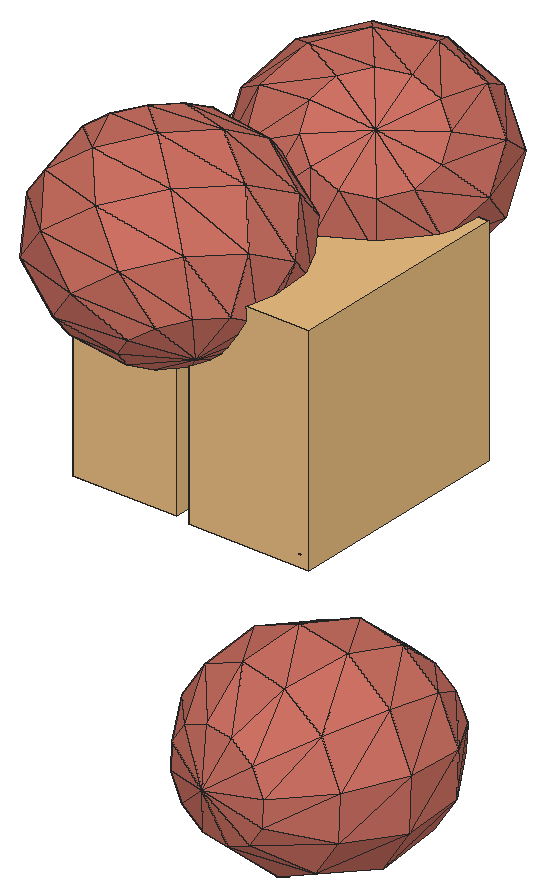
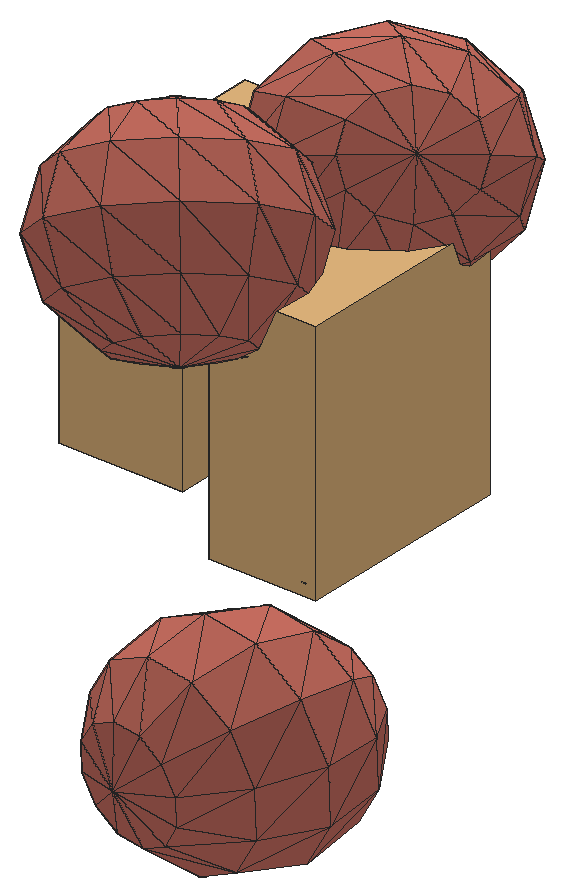
# SketchUp Ruby script. Lengths in inches.
U = 1.inch
M = Sketchup.active_model
def pt(a) = Geom::Point3d.new(a.map { |v| v * U })
def face(e, loops, mat)
  f = e.add_face(loops[0].map { |a| pt(a) })
  loops[1..].each { |l| e.add_face(l.map { |a| pt(a) }).erase! }
  f.material = f.back_material = mat if mat
  f
end
# faces: each face lists its corners as indices into pts; further lists are holes
def faces(e, pts, list, mat = nil) = list.each { |f| face(e, (f[0].is_a?(Array) ? f : [f]).map { |l| l.map { |i| pts[i] } }, mat) }
# xy, xz, yz: faces in a plane at the given z, y or x. An outline is a flat list of corners, or four numbers for a rectangle; further outlines are holes
def ring(l) = l.size == 4 ? [[l[0], l[1]], [l[2], l[1]], [l[2], l[3]], [l[0], l[3]]] : l.each_slice(2).to_a
def flat(e, list, mat, &to3) = list.each { |f| face(e, (f[0].is_a?(Array) ? f : [f]).map { |l| ring(l).map { |u, v| to3.(u, v) } }, mat) }
def xy(e, z, list, mat = nil) = flat(e, list, mat) { |x, y| [x, y, z] }
def xz(e, y, list, mat = nil) = flat(e, list, mat) { |x, z| [x, y, z] }
def yz(e, x, list, mat = nil) = flat(e, list, mat) { |y, z| [x, y, z] }
def lines(e, pts, list) = list.each { |a, b| e.add_line(pt(pts[a]), pt(pts[b])) }
# prism: a flat outline (further loops are holes) pulled along v
def prism(e, loops, v, mat = nil)
  f = face(e, loops, mat); d = Geom::Vector3d.new(v.map { |x| x * U })
  f.pushpull(f.normal.samedirection?(d) ? d.length : -d.length)
end
def box(e, o, s, mat = nil) = prism(e, [[o, [o[0] + s[0], o[1], o[2]], [o[0] + s[0], o[1] + s[1], o[2]], [o[0], o[1] + s[1], o[2]]]], [0, 0, s[2]], mat)
def at(x, y, z, deg = 0) = Geom::Transformation.translation(pt([x, y, z])) * Geom::Transformation.rotation(ORIGIN, Z_AXIS, deg.degrees)
def axes(o, x, y, z) = Geom::Transformation.new([*x, 0, *y, 0, *z, 0, *pt(o).to_a, 1])
def part(name) = M.definitions.add(name)
# library, detail: a bought-in or finely detailed component or shape, given as its bounding box
def library(name, o, s) = part(name).tap { |d| box(d.entities, o, s) }
def detail(e, o, s) = box(e.add_group.entities, o, s)
def put(e, d, t, mat = nil) = e.add_instance(d, t).tap { |i| i.material = mat if mat }
def group(e, t, mat = nil) = e.add_group.tap { |g| g.transformation = t; g.material = mat if mat }.entities
root = M.entities
M.materials.add("green").color = [174, 139, 102]
M.materials.add("vio").color = [206, 114, 100]
c1 = library("3DGeom~152_Defintion",[-440.97,-500,-219.08],[881.94,1000,438.17])
c2 = part("3DGeom~153_Defintion")
p = [[-380.69,-485.53,-210.54],[-411.26,-467,-218.1875],[-394.16,-475.51,-219.08],[-380.69,-485.53,-210.54],[-434.74,-476.74,-157.14],[-411.26,-467,-218.1875],
  [-438.29,-462.61,-191.49],[-411.26,-467,-218.1875],[-438.29,-462.61,-191.49],[-427.41,-462.28,-208.09],[-377.14,-499.67,-176.1875],[-434.74,-476.74,-157.14],
  [-380.69,-485.53,-210.54],[-377.14,-499.67,-176.1875],[-380.69,-485.53,-210.54],[-374.46,-494.375,-194.84],[-434.74,-476.74,-157.14],[-440.97,-467.9,-172.84],
  [-438.29,-462.61,-191.49],[-404.17,-495.28,-149.49],[-377.14,-499.67,-176.1875],[-388.02,-500,-159.59],[-404.17,-495.28,-149.49],[-434.74,-476.74,-157.14],
  [-404.17,-495.28,-149.49],[-421.27,-486.76,-148.59],[402.51,492.03,208.37],[431.04,458.58,149.1],[419.28,470.25,140.95],[402.51,492.03,208.37],
  [419.28,470.25,140.95],[406.85,483.28,142.92],[402.51,492.03,208.37],[406.85,483.28,142.92],[397.08,494.16,154.49],[402.51,492.03,208.37],
  [438.98,451.39,165.19],[431.04,458.58,149.1],[402.51,492.03,208.37],[397.08,494.16,154.49],[392.58,500,172.55],[402.51,492.03,208.37],
  [440.97,450.61,184.92],[438.98,451.39,165.19],[402.51,492.03,208.37],[392.58,500,172.55],[394.57,499.22,192.28],[402.51,492.03,208.37],
  [436.48,456.44,202.98],[440.97,450.61,184.92],[402.51,492.03,208.37],[426.7,467.33,214.55],[402.51,492.03,208.37],[414.27,480.36,216.53],
  [426.7,467.33,214.55]]
faces(c2.entities,p,[[0,1,2],[3,4,5],[5,4,6],[7,8,9],[10,11,12],[13,14,15],[16,17,18],[19,20,21],
  [22,11,10],[23,24,25],[26,27,28],[29,30,31],[32,33,34],[35,36,37],[38,39,40],[41,42,43],
  [44,45,46],[47,48,49],[50,51,48],[52,53,54]],"green")
c3 = part("3DGeom~238_Defintion")
p = [[47.04,-55.62,-493.71],[-13.56,-317.59,-331.8],[-140.27,-151.99,-445.55],[202.73,-206.32,-387.4],[187.3,88.625,-451.96],[-121.25,109.98,-467.72],
  [-40.27,193.26,-443.62],[-229.4,54.34,-439.92],[-257.06,246.11,-316.41],[364.69,-39.76,-339.2],[242.94,242.1,-331.5],[-8.15,281.87,-374.07],
  [-226.21,-343.77,-187.29],[-324.43,-174.66,-320.41],[-335.72,41.26,-367.67],[202.73,-206.32,-387.4],[116.79,-398.1,-129.14],[-13.56,-317.59,-331.8],
  [202.73,-206.32,-387.4],[304.09,-301.73,-177.3],[364.69,-39.76,-339.2],[304.09,-301.73,-177.3],[202.73,-206.32,-387.4],[-33.49,352.06,-277.72],
  [242.94,242.1,-331.5],[-8.15,281.87,-374.07],[-33.49,352.06,-277.72],[-335.72,41.26,-367.67],[-324.43,-174.66,-320.41],[-456.1,-117.55,-151.8],
  [-335.72,41.26,-367.67],[-411.74,74.22,-270.32],[-335.72,41.26,-367.67],[-257.06,246.11,-316.41],[364.69,-39.76,-339.2],[444.36,-157.49,-135.55],
  [304.09,-301.73,-177.3],[428.9375,137.45,-200.11],[364.69,-39.76,-339.2],[428.9375,137.45,-200.11],[-13.56,-317.59,-331.8],[-67.38,-420.77,-4],
  [-226.21,-343.77,-187.29],[-13.56,-317.59,-331.8],[199.05,363.67,-164.61],[428.9375,137.45,-200.11],[242.94,242.1,-331.5],[-33.49,352.06,-277.72],
  [199.05,363.67,-164.61],[242.94,242.1,-331.5],[-324.43,-174.66,-320.41],[-226.21,-343.77,-187.29],[-378.25,-277.83,7.4],[-324.43,-174.66,-320.41],
  [-437.09,144.42,-173.96],[-257.06,246.11,-316.41],[-404.96,233.02,-104.42],[-257.06,246.11,-316.41],[-323.98,316.3,-80.32],[-257.06,246.11,-316.41],
  [-323.98,316.3,-80.32],[-215.84,371.9375,-108.12],[-257.06,246.11,-316.41],[-109.51,385.02,-180.37],[-33.49,352.06,-277.72],[-257.06,246.11,-316.41],
  [-257.06,246.11,-316.41],[-33.49,352.06,-277.72],[-500,4.02,15.09],[428.9375,137.45,-200.11],[500,-4.02,-15.09],[378.25,277.83,-7.4],
  [428.9375,137.45,-200.11],[199.05,363.67,-164.61],[428.9375,137.45,-200.11],[-226.21,-343.77,-187.29],[-199.05,-363.67,164.61],[-226.21,-343.77,-187.29],
  [-199.05,-363.67,164.61],[-378.25,-277.83,7.4],[67.38,420.77,4],[215.84,-371.9375,108.12],[323.98,-316.3,80.32],[323.98,-316.3,80.32],
  [304.09,-301.73,-177.3],[-444.36,157.49,135.55],[378.25,277.83,-7.4],[-428.9375,-137.45,200.11],[404.96,-233.02,104.42],[323.98,-316.3,80.32],
  [109.51,-385.02,180.37],[-116.78,398.1,129.14],[-304.09,301.73,177.3],[-304.09,301.73,177.3],[-323.98,316.3,-80.32],[-304.09,301.73,177.3],
  [437.09,-144.42,173.96],[456.1,117.55,151.8],[226.21,343.77,187.29],[226.21,343.77,187.29],[378.25,277.83,-7.4],[33.49,-352.06,277.72],
  [-199.05,-363.67,164.61],[-199.05,-363.67,164.61],[-242.94,-242.09,331.5],[-242.94,-242.09,331.5],[-364.69,39.76,339.2],[257.06,-246.11,316.41],
  [323.98,-316.3,80.32],[257.06,-246.11,316.41],[257.06,-246.11,316.41],[13.56,317.59,331.8],[-202.73,206.32,387.4],[-202.73,206.32,387.4],
  [-304.09,301.73,177.3],[411.74,-74.22,270.32],[324.43,174.66,320.41],[226.21,343.77,187.29],[-199.05,-363.67,164.61],[8.15,-281.87,374.07],
  [-242.94,-242.09,331.5],[-199.05,-363.67,164.61],[8.15,-281.87,374.07],[257.06,-246.11,316.41],[-202.73,206.32,387.4],[13.56,317.59,331.8],
  [324.43,174.66,320.41],[226.21,343.77,187.29],[-428.9375,-137.45,200.11],[-242.94,-242.09,331.5],[-187.3,-88.625,451.96],[-428.9375,-137.45,200.11],
  [-364.69,39.76,339.2],[335.72,-41.26,367.67],[257.06,-246.11,316.41],[8.15,-281.87,374.07],[33.49,-352.06,277.72],[257.06,-246.11,316.41],
  [40.27,-193.26,443.62],[257.06,-246.11,316.41],[121.25,-109.98,467.72],[257.06,-246.11,316.41],[229.4,-54.34,439.92],[257.06,-246.11,316.41],
  [335.72,-41.26,367.67],[257.06,-246.11,316.41],[140.27,151.99,445.55],[335.72,-41.26,367.67],[324.43,174.66,320.41],[13.56,317.59,331.8],
  [324.43,174.66,320.41],[-202.73,206.32,387.4],[13.56,317.59,331.8],[-364.69,39.76,339.2],[-47.04,55.62,493.71],[-364.69,39.76,339.2],
  [-202.73,206.32,387.4],[335.72,-41.26,367.67],[-202.73,206.32,387.4]]
faces(c3.entities,p,[[0,1,2],[0,3,1],[4,3,0],[5,0,2],[6,0,5],[6,4,0],[5,2,7],[5,7,8],
  [6,5,8],[4,9,3],[10,9,4],[11,4,6],[11,10,4],[2,12,13],[2,1,12],[7,2,13],
  [11,6,8],[7,13,14],[7,14,8],[15,16,17],[18,19,16],[20,21,22],[23,24,25],[26,11,8],
  [27,28,29],[30,29,31],[32,31,33],[34,35,36],[37,35,38],[10,39,9],[40,41,42],[43,16,41],
  [44,45,46],[47,48,49],[50,51,52],[53,52,29],[31,54,55],[54,56,57],[56,58,59],[60,61,62],
  [63,64,65],[61,63,66],[63,48,67],[31,29,68],[31,68,54],[69,70,35],[71,70,72],[73,71,74],
  [75,41,76],[77,78,79],[63,80,48],[61,80,63],[19,81,16],[19,82,81],[35,83,84],[54,68,85],
  [54,85,56],[80,86,48],[29,52,87],[29,87,68],[35,88,89],[70,88,35],[16,90,41],[16,81,90],
  [60,91,61],[61,91,80],[56,85,92],[56,93,94],[60,95,91],[70,96,88],[97,96,70],[71,97,70],
  [98,97,71],[80,99,100],[41,101,102],[41,90,101],[91,99,80],[52,103,104],[52,105,87],[68,87,106],
  [68,106,85],[81,82,107],[108,88,109],[88,96,110],[90,81,107],[95,111,91],[91,111,99],[85,106,112],
  [85,113,114],[97,115,96],[116,115,97],[117,116,97],[118,119,120],[121,101,122],[96,115,123],[95,124,111],
  [101,90,107],[125,126,127],[128,129,130],[131,130,132],[115,133,134],[116,133,115],[135,136,137],[138,135,139],
  [140,138,141],[142,140,143],[144,142,145],[146,147,148],[149,146,150],[129,135,138],[129,138,130],[151,146,152],
  [153,130,154],[155,154,156],[146,142,157],[158,154,146],[154,140,142],[154,142,146],[130,138,140],[130,140,154]],"vio")
c4 = part("3DGeom~206_Defintion")
p = [[-12.5,-12.78,-500],[-167.87,-176.1875,-423.23],[-275,-119.8,-393.5],[139.12,-146.19,-448.74],[321.29,0,-383.61],[-198.05,84.89,-448.51],
  [146.22,154.06,-442.79],[216.18,-279.61,-308.47],[-80.33,-253.22,-393.64],[410.28,-154.06,-221.63],[410.28,-154.06,-221.63],[-373.01,-99.16,-312.41],
  [-373.01,-99.16,-312.41],[-367.81,120.64,-308.0625],[-68.03,266.84,-383.34],[-367.81,120.64,-308.0625],[-68.03,266.84,-383.34],[417.375,146.19,-215.68],
  [417.375,146.19,-215.68],[265.76,279.61,-266.94],[265.76,279.61,-266.94],[-68.03,266.84,-383.34],[-278.26,-292.39,-233.06],[-278.26,-292.39,-233.06],
  [-35.84,-330.25,-312.65],[-278.26,-292.39,-233.06],[-373.01,-99.16,-312.41],[-275,-119.8,-393.5],[-278.26,-292.39,-233.06],[494.4375,12.78,-75.41],
  [410.28,-154.06,-221.63],[321.29,0,-383.61],[321.29,0,-383.61],[417.375,146.19,-215.68],[-68.03,266.84,-383.34],[-367.81,120.64,-308.0625],
  [-264.06,308.11,-221.16],[80.21,377.28,-215.45],[-68.03,266.84,-383.34],[-264.06,308.11,-221.16],[265.76,279.61,-266.94],[-68.03,266.84,-383.34],
  [80.21,377.28,-215.45],[-35.84,-330.25,-312.65],[-46.32,-386.64,-201.97],[-278.26,-292.39,-233.06],[198.04,-377.28,-116.76],[-35.84,-330.25,-312.65],
  [198.04,-377.28,-116.76],[-35.84,-330.25,-312.65],[216.18,-279.61,-308.47],[-435.64,-119.8,-201.7],[-278.26,-292.39,-233.06],[-367.81,120.64,-308.0625],
  [389.33,-266.84,-0.27],[198.04,-377.28,-116.76],[216.18,-279.61,-308.47],[216.18,-279.61,-308.47],[-476.3,84.89,-116.29],[-264.06,308.11,-221.16],
  [401.625,253.22,10.03],[265.76,279.61,-266.94],[265.76,279.61,-266.94],[314.09,330.25,-19.5625],[314.09,330.25,-19.5625],[265.76,279.61,-266.94],
  [-108.95,-407.27,-91.25],[-206.96,-386.64,-10.17],[-314.09,-330.25,19.5625],[-314.09,-330.25,19.5625],[-401.625,-253.22,-10.03],[-278.26,-292.39,-233.06],
  [-446.12,-176.1875,-91.02],[-278.26,-292.39,-233.06],[-278.26,-292.39,-233.06],[476.3,-84.89,116.29],[-264.06,308.11,-221.16],[-389.33,266.84,0.27],
  [-89.55,413.03,-75],[-389.33,266.84,0.27],[446.12,176.1875,91.02],[206.96,386.64,10.17],[89.55,-413.03,75],[198.04,-377.28,-116.76],
  [264.06,-308.11,221.16],[198.04,-377.28,-116.76],[264.06,-308.11,221.16],[198.04,-377.28,-116.76],[389.33,-266.84,-0.27],[-494.4375,-12.78,75.41],
  [-80.21,-377.28,215.45],[435.64,119.8,201.7],[-389.33,266.84,0.27],[-198.04,377.28,116.76],[108.95,407.27,91.25],[314.09,330.25,-19.5625],
  [278.26,292.39,233.06],[278.26,292.39,233.06],[-265.76,-279.61,266.94],[-265.76,-279.61,266.94],[-417.375,-146.19,215.68],[-314.09,-330.25,19.5625],
  [-417.375,-146.19,215.68],[367.81,-120.64,308.0625],[264.06,-308.11,221.16],[367.81,-120.64,308.0625],[-410.28,154.06,221.63],[-198.04,377.28,116.76],
  [-410.28,154.06,221.63],[278.26,292.39,233.06],[-417.375,-146.19,215.68],[-314.09,-330.25,19.5625],[-265.76,-279.61,266.94],[68.03,-266.84,383.34],
  [68.03,-266.84,383.34],[264.06,-308.11,221.16],[-410.28,154.06,221.63],[-417.375,-146.19,215.68],[46.32,386.64,201.97],[278.26,292.39,233.06],
  [373.01,99.16,312.41],[367.81,-120.64,308.0625],[-198.04,377.28,116.76],[-410.28,154.06,221.63],[-216.18,279.61,308.47],[-216.18,279.61,308.47],
  [-216.18,279.61,308.47],[35.84,330.25,312.65],[35.84,330.25,312.65],[278.26,292.39,233.06],[-146.22,-154.06,442.79],[-265.76,-279.61,266.94],
  [-80.21,-377.28,215.45],[-80.21,-377.28,215.45],[68.03,-266.84,383.34],[-321.29,0,383.61],[-417.375,-146.19,215.68],[-410.28,154.06,221.63],
  [-417.375,-146.19,215.68],[-321.29,0,383.61],[198.05,-84.89,448.51],[264.06,-308.11,221.16],[367.81,-120.64,308.0625],[-216.18,279.61,308.47],
  [-410.28,154.06,221.63],[275,119.8,393.5],[167.87,176.1875,423.23],[275,119.8,393.5],[278.26,292.39,233.06],[80.33,253.22,393.64],
  [278.26,292.39,233.06],[35.84,330.25,312.65],[278.26,292.39,233.06],[275,119.8,393.5],[275,119.8,393.5],[373.01,99.16,312.41],
  [-139.12,146.19,448.74],[12.5,12.78,500],[275,119.8,393.5]]
faces(c4.entities,p,[[0,1,2],[3,1,0],[4,3,0],[0,2,5],[6,0,5],[4,0,6],[7,8,3],[9,7,3],
  [3,8,1],[10,3,4],[5,2,11],[5,12,13],[14,5,15],[6,5,16],[17,4,6],[18,6,19],
  [20,6,21],[2,1,22],[1,8,23],[8,24,25],[7,24,8],[26,27,28],[29,30,31],[29,32,33],
  [34,35,36],[37,38,39],[40,41,42],[43,44,45],[46,44,47],[48,49,50],[51,26,52],[53,26,51],
  [54,55,56],[54,57,30],[53,51,58],[59,53,58],[60,33,61],[60,62,63],[64,65,37],[66,67,45],
  [44,66,45],[67,68,45],[69,70,71],[70,72,73],[72,51,74],[75,54,30],[75,30,29],[76,58,77],
  [78,39,79],[37,39,78],[80,29,33],[80,33,60],[64,37,81],[81,37,78],[82,66,44],[82,44,83],
  [58,51,72],[84,82,85],[86,87,88],[58,72,89],[77,58,89],[90,66,82],[90,67,66],[89,72,70],
  [91,75,29],[91,29,80],[78,92,93],[94,78,93],[81,78,94],[60,95,96],[64,81,97],[98,68,67],
  [99,67,90],[100,70,101],[89,70,102],[103,104,54],[105,54,75],[77,89,106],[107,77,108],[80,60,96],
  [81,94,109],[110,111,112],[113,90,82],[114,82,115],[116,89,117],[91,80,96],[94,118,119],[94,93,118],
  [120,121,75],[120,75,91],[122,123,124],[118,93,125],[120,91,96],[118,126,127],[118,128,129],[130,131,132],
  [130,133,134],[135,136,131],[137,138,139],[140,134,141],[140,141,142],[143,144,135],[145,120,96],[146,147,148],
  [149,146,150],[151,149,152],[135,131,130],[153,140,142],[154,142,155],[143,135,156],[151,143,156],[151,156,149],
  [157,130,134],[157,134,140],[156,135,130],[146,140,158],[149,156,157],[149,157,146],[146,157,140],[156,130,157]],"vio")
c5 = part("3DGeom~199_Defintion")
p = [[-69.55,-302.43,-360.84],[-338.74,-97.12,-366.25],[-102.46,-106.03,-485.67],[189.77,-256.61,-366.85],[161.26,-86.52,-474.95],[-343.46,97.57,-361.65],
  [-107.92,118.79,-480.36],[156.54,108.18,-470.35],[-323.15,264.7,-245.58],[-84.47,311.77,-346.33],[-323.15,264.7,-245.58],[-84.47,311.77,-346.33],
  [398.24,-142.03,-274.56],[398.24,-142.03,-274.56],[381.78,-43.83,-336.97],[381.78,-43.83,-336.97],[381.78,-43.83,-336.97],[379.05,68.57,-334.3125],
  [379.05,68.57,-334.3125],[176.85,275.3,-354.28],[-84.47,311.77,-346.33],[176.85,275.3,-354.28],[234.41,-356.52,-175.01],[-69.55,-302.43,-360.84],
  [189.77,-256.61,-366.85],[424.01,-199.72,-163.8],[234.41,-356.52,-175.01],[189.77,-256.61,-366.85],[189.77,-256.61,-366.85],[398.24,-142.03,-274.56],
  [-310.23,-267.21,-258.15],[-310.23,-267.21,-258.15],[-484.24,-62.19,-148.7],[-338.74,-97.12,-366.25],[-338.74,-97.12,-366.25],[-486.97,50.21,-146.04],
  [-338.74,-97.12,-366.25],[-343.46,97.57,-361.65],[-343.46,97.57,-361.65],[-475.25,146.71,-79.03],[-343.46,97.57,-361.65],[-323.15,264.7,-245.58],
  [-18,-417.8,-139.33],[-310.23,-267.21,-258.15],[-69.55,-302.43,-360.84],[234.41,-356.52,-175.01],[-69.55,-302.43,-360.84],[379.05,68.57,-334.3125],
  [176.85,275.3,-354.28],[390.78,165.07,-267.3],[390.78,165.07,-267.3],[176.85,275.3,-354.28],[216.77,370.09,-157.85],[176.85,275.3,-354.28],
  [-84.47,311.77,-346.33],[-38.375,421.22,-119.51],[176.85,275.3,-354.28],[216.77,370.09,-157.85],[-323.15,264.7,-245.58],[-283.23,359.48,-49.15],
  [381.78,-43.83,-336.97],[500,10.6,-108.7],[379.05,68.57,-334.3125],[413.82,219.79,-153.89],[-265.59,-367.12,-66.32],[-310.23,-267.21,-258.15],
  [-265.59,-367.12,-66.32],[-467.79,-160.39,-86.29],[-310.23,-267.21,-258.15],[-310.23,-267.21,-258.15],[-323.15,264.7,-245.58],[-452.2,201.43,34.38],
  [-323.15,264.7,-245.58],[-283.23,359.48,-49.15],[283.23,-359.48,49.15],[234.41,-356.52,-175.01],[452.2,-201.43,-34.38],[283.23,-359.48,49.15],
  [265.59,367.12,66.32],[216.77,370.09,-157.85],[18,417.8,139.33],[265.59,367.12,66.32],[216.77,370.09,-157.85],[442.01,218.08,-24.47],
  [-500,-10.6,108.7],[38.375,-421.22,119.51],[283.23,-359.48,49.15],[-234.41,356.52,175.02],[475.25,-146.71,79.03],[486.97,-50.21,146.04],
  [484.24,62.19,148.7],[467.79,160.39,86.29],[-265.59,-367.12,-66.32],[-442.01,-218.08,24.47],[-216.77,-370.09,157.85],[-216.77,-370.09,157.85],
  [-265.59,-367.12,-66.32],[-283.23,359.48,-49.15],[-424.01,199.72,163.8],[-283.23,359.48,-49.15],[-234.41,356.52,175.02],[310.23,267.21,258.15],
  [-216.77,-370.09,157.85],[-413.82,-219.79,153.89],[323.15,-264.7,245.59],[283.23,-359.48,49.15],[323.15,-264.7,245.59],[265.59,367.12,66.32],
  [69.55,302.43,360.84],[310.23,267.21,258.15],[265.59,367.12,66.32],[69.55,302.43,360.84],[338.74,97.12,366.25],[-390.78,-165.07,267.3],
  [-390.78,-165.07,267.3],[-379.05,-68.57,334.3125],[-379.05,-68.57,334.3125],[-381.78,43.83,336.97],[-381.78,43.83,336.97],[-398.24,142.03,274.56],
  [-398.24,142.03,274.56],[84.47,-311.77,346.34],[323.15,-264.7,245.59],[84.47,-311.77,346.34],[-189.77,256.61,366.85],[-189.77,256.61,366.85],
  [69.55,302.43,360.84],[343.46,-97.57,361.65],[-176.85,-275.3,354.28],[-216.77,-370.09,157.85],[-176.85,-275.3,354.28],[-390.78,-165.07,267.3],
  [84.47,-311.77,346.34],[-176.85,-275.3,354.28],[-234.41,356.52,175.02],[-398.24,142.03,274.56],[-234.41,356.52,175.02],[-398.24,142.03,274.56],
  [-189.77,256.61,366.85],[343.46,-97.57,361.65],[84.47,-311.77,346.34],[323.15,-264.7,245.59],[310.23,267.21,258.15],[102.46,106.03,485.67],
  [338.74,97.12,366.25],[310.23,267.21,258.15],[69.55,302.43,360.84],[-156.54,-108.17,470.35],[-390.78,-165.07,267.3],[-176.85,-275.3,354.28],
  [-379.05,-68.57,334.3125],[-189.77,256.61,366.85],[-398.24,142.03,274.56],[-381.78,43.83,336.97],[-161.26,86.52,474.95],[107.92,-118.79,480.36],
  [343.46,-97.57,361.65],[338.74,97.12,366.25],[343.46,-97.57,361.65],[338.74,97.12,366.25]]
faces(c5.entities,p,[[0,1,2],[3,0,2],[3,2,4],[2,1,5],[2,5,6],[4,2,6],[4,6,7],[6,5,8],
  [7,6,9],[6,10,11],[12,3,4],[13,4,14],[15,4,7],[16,7,17],[18,7,19],[7,20,21],
  [22,23,24],[25,26,27],[25,28,29],[0,30,1],[31,32,33],[34,32,35],[36,35,37],[38,35,39],
  [40,39,41],[42,43,44],[45,42,46],[47,48,49],[50,51,52],[53,54,55],[56,55,57],[54,58,59],
  [54,59,55],[29,60,61],[60,62,61],[62,50,61],[25,29,61],[50,63,61],[50,52,63],[42,64,65],
  [66,67,68],[69,67,32],[70,39,71],[72,71,73],[74,42,75],[76,77,26],[76,26,25],[76,25,61],
  [63,52,78],[79,80,81],[82,55,80],[63,83,61],[63,78,83],[32,67,84],[35,32,84],[39,35,84],
  [85,64,42],[86,85,42],[55,59,87],[55,87,80],[88,76,61],[89,88,61],[90,89,61],[83,91,61],
  [91,90,61],[92,93,67],[67,93,84],[71,39,84],[85,94,64],[95,93,96],[97,71,98],[99,98,100],
  [88,77,76],[83,101,91],[83,78,101],[102,103,93],[93,103,84],[98,71,84],[104,85,105],[88,106,77],
  [107,108,109],[110,80,111],[89,106,88],[91,112,90],[91,101,112],[103,113,84],[114,115,84],[116,117,84],
  [118,119,84],[120,98,84],[121,94,85],[122,123,85],[80,87,124],[80,125,126],[89,127,106],[90,127,89],
  [90,112,127],[128,103,129],[130,131,103],[132,133,94],[134,98,135],[136,137,138],[139,140,141],[142,143,144],
  [145,146,143],[147,148,149],[147,150,148],[151,152,153],[154,150,147],[154,153,150],[151,153,154],[155,149,140],
  [156,155,140],[155,147,149],[146,151,154],[146,154,143],[157,155,158],[159,143,155],[143,147,155],[143,154,147]],"vio")
c6 = library("3DGeom~61_Defintion",[-500,-478.45,-265.375],[1000,956.89,530.75])
c7 = part("3DGeom~62_Defintion")
p = [[-465.47,464.9,-258.6875],[-477.89,451.53,-263.24],[-489.74,438.22,-257.15],[-465.47,464.9,-258.6875],[-497.83,428.53,-242.0625],[-500,425.07,-222.01],
  [-465.47,464.9,-258.6875],[-500,425.07,-222.01],[-495.67,428.76,-202.375],[-465.47,464.9,-258.6875],[-489.74,438.22,-257.15],[-497.83,428.53,-242.0625],
  [-465.47,464.9,-258.6875],[-495.67,428.76,-202.375],[-485.99,438.61,-188.41],[-465.47,464.9,-258.6875],[-485.99,438.61,-188.41],[-473.5625,451.98,-183.86],
  [-465.47,464.9,-258.6875],[-473.5625,451.98,-183.86],[-461.72,465.3,-189.95],[-465.47,464.9,-258.6875],[-453.625,474.98,-205.04],[-451.46,478.44,-225.09],
  [-465.47,464.9,-258.6875],[-451.46,478.44,-225.09],[-455.79,474.75,-244.72],[-465.47,464.9,-258.6875],[-461.72,465.3,-189.95],[-453.625,474.98,-205.04],
  [492.22,-453.97,197.65],[460.87,-474.71,197.28],[477.9,-465.75,192.59],[460.87,-474.71,197.28],[436.46,-475.96,228.62],[445.7,-478.45,210.47],
  [460.87,-474.71,197.28],[492.22,-453.97,197.65],[436.46,-475.96,228.62],[436.46,-475.96,228.62],[492.22,-453.97,197.65],[443.4,-456.48,260.3125],
  [443.4,-456.48,260.3125],[492.22,-453.97,197.65],[474.74,-435.74,260.68],[474.74,-435.74,260.68],[492.22,-453.97,197.65],[499.15,-434.48,229.35],
  [492.22,-453.97,197.65],[500,-442.52,211.1],[499.15,-434.48,229.35],[436.46,-475.96,228.62],[443.4,-456.48,260.3125],[435.62,-467.92,246.86],
  [474.74,-435.74,260.68],[499.15,-434.48,229.35],[489.91,-432,247.49],[443.4,-456.48,260.3125],[474.74,-435.74,260.68],[457.72,-444.7,265.375]]
faces(c7.entities,p,[[0,1,2],[3,4,5],[6,7,8],[9,10,11],[12,13,14],[15,16,17],[18,19,20],[21,22,23],
  [24,25,26],[27,28,29],[30,31,32],[33,34,35],[36,37,38],[39,40,41],[42,43,44],[45,46,47],
  [48,49,50],[51,52,53],[54,55,56],[57,58,59]],"green")
g1 = group(root,at(15.3125,134.49,26.21))
put(g1,c1,axes([-1.7,0.38,12.49],[0,0.00039,0],[0,0,-0.00039],[-0.00039,0,0]),"green")
put(g1,c2,axes([-1.7,0.38,12.49],[0,0.00039,0],[0,0,-0.00039],[-0.00039,0,0]),"green")
g2 = group(root,at(15.3125,134.49,26.21))
put(g2,c3,axes([-1.62,0.2,12.71],[0,0.00039,0],[0,0,-0.00039],[-0.00039,0,0]),"vio")
g3 = group(root,at(15.3125,134.49,26.21))
put(g3,c4,axes([-1.54,0.52,12.72],[0,0.00039,0],[0,0,-0.00039],[-0.00039,0,0]),"vio")
g4 = group(root,at(15.3125,134.49,26.21))
put(g4,c5,axes([-1.51,0.37,11.92],[0,0.00038,0],[0,0,-0.00038],[-0.00038,0,0]),"vio")
g5 = group(root,at(15.3125,134.49,26.21))
put(g5,c6,axes([-1.4375,0.32,12.52],[0,0.00037,0],[0,0,-0.00037],[-0.00037,0,0]),"green")
put(g5,c7,axes([-1.4375,0.32,12.52],[0,0.00037,0],[0,0,-0.00037],[-0.00037,0,0]),"green")
